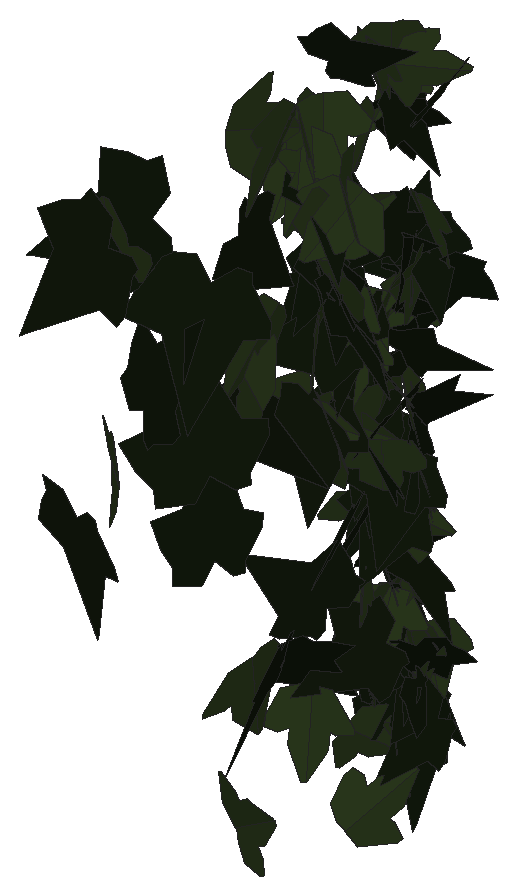
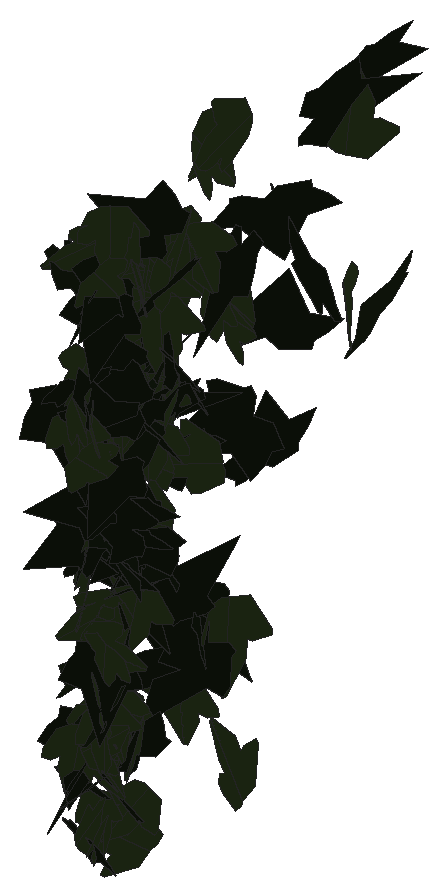
# SketchUp Ruby script. Lengths in inches.
U = 1.inch
M = Sketchup.active_model
def pt(a) = Geom::Point3d.new(a.map { |v| v * U })
def face(e, loops, mat)
  f = e.add_face(loops[0].map { |a| pt(a) })
  loops[1..].each { |l| e.add_face(l.map { |a| pt(a) }).erase! }
  f.material = f.back_material = mat if mat
  f
end
# faces: each face lists its corners as indices into pts; further lists are holes
def faces(e, pts, list, mat = nil) = list.each { |f| face(e, (f[0].is_a?(Array) ? f : [f]).map { |l| l.map { |i| pts[i] } }, mat) }
# xy, xz, yz: faces in a plane at the given z, y or x. An outline is a flat list of corners, or four numbers for a rectangle; further outlines are holes
def ring(l) = l.size == 4 ? [[l[0], l[1]], [l[2], l[1]], [l[2], l[3]], [l[0], l[3]]] : l.each_slice(2).to_a
def flat(e, list, mat, &to3) = list.each { |f| face(e, (f[0].is_a?(Array) ? f : [f]).map { |l| ring(l).map { |u, v| to3.(u, v) } }, mat) }
def xy(e, z, list, mat = nil) = flat(e, list, mat) { |x, y| [x, y, z] }
def xz(e, y, list, mat = nil) = flat(e, list, mat) { |x, z| [x, y, z] }
def yz(e, x, list, mat = nil) = flat(e, list, mat) { |y, z| [x, y, z] }
def lines(e, pts, list) = list.each { |a, b| e.add_line(pt(pts[a]), pt(pts[b])) }
# prism: a flat outline (further loops are holes) pulled along v
def prism(e, loops, v, mat = nil)
  f = face(e, loops, mat); d = Geom::Vector3d.new(v.map { |x| x * U })
  f.pushpull(f.normal.samedirection?(d) ? d.length : -d.length)
end
def box(e, o, s, mat = nil) = prism(e, [[o, [o[0] + s[0], o[1], o[2]], [o[0] + s[0], o[1] + s[1], o[2]], [o[0], o[1] + s[1], o[2]]]], [0, 0, s[2]], mat)
def at(x, y, z, deg = 0) = Geom::Transformation.translation(pt([x, y, z])) * Geom::Transformation.rotation(ORIGIN, Z_AXIS, deg.degrees)
def axes(o, x, y, z) = Geom::Transformation.new([*x, 0, *y, 0, *z, 0, *pt(o).to_a, 1])
def part(name) = M.definitions.add(name)
# library, detail: a bought-in or finely detailed component or shape, given as its bounding box
def library(name, o, s) = part(name).tap { |d| box(d.entities, o, s) }
def detail(e, o, s) = box(e.add_group.entities, o, s)
def put(e, d, t, mat = nil) = e.add_instance(d, t).tap { |i| i.material = mat if mat }
def group(e, t, mat = nil) = e.add_group.tap { |g| g.transformation = t; g.material = mat if mat }.entities
root = M.entities
M.materials.add("efeu1").color = [18, 25, 13]
M.materials.add("efeu2").color = [43, 57, 29]
c1 = part("ivyleaf_9")
p = [[1.54,2.16,1.25],[1.36,2.04,1.19],[-0.21,0.99,0.68],[-0.71,1.11,0.82],[-0.85,0.86,0.67],[-0.8,0.17,0.21],
  [-0.9,-0.01,0.1],[-0.67,-0.16,-0.02],[-0.08,-0.08,-0.05],[-0.03,-0.6,-0.4],[0.65,-0.88,-0.66],[0.83,-0.6,-0.49],
  [1.29,-0.42,-0.43],[1.8125,-0.07,-0.26],[1.21,0.44,0.15]]
faces(c1.entities,p,[[0,1,2,3,4,5,6,7,8,9,10,11,12,13,14]],"efeu1")
c2 = part("ivyleaf_10")
p = [[0,0.5,-0.03],[-0.0625,2.02,-0.43],[-0.19,2.01,-0.46],[-0.54,1.05,-0.29],[-0.52,0.625,-0.18],[-0.83,0.76,-0.28],
  [-1.16,0.64,-0.33],[-1.15,0.33,-0.24],[-0.77,-0.39,0.02],[-0.3,-0.51,0.16],[0.04,-0.48,0.23],[-0.02,2.01,-0.4375],
  [-0.06,2.01,-0.43],[0.04,-0.49,0.23],[0.67,-0.49,0.14],[1.38,0.36,-0.2],[1.375,0.51,-0.24],[0.81,0.65,-0.19],
  [0.62,0.59,-0.15],[0.6,1.09,-0.28],[0.5,1.23,-0.31]]
faces(c2.entities,p,[[0,1,2,3,4,5,6,7,8,9,10],[11,12,0,13,14,15,16,17,18,19,20]],"efeu2")
put(root,c1,axes([600.29,122.28,205.0625],[-0.40214,-0.86547,0.79158],[-0.29941,-0.73333,-0.9539],[1.13401,-0.50053,0.02885]))
put(root,c1,axes([599.61,122.04,197.19],[0.37416,-1.0394,0.54489],[0.18019,-0.51425,-1.10469],[1.15965,0.41527,-0.00415]))
put(root,c2,axes([599.48,123.61,203.85],[-1.04539,-0.23981,-0.03283],[-0.02592,-0.03381,1.0722],[-0.24065,1.04536,0.02715]))
put(root,c1,axes([599.8,124.59,204.78],[-0.4061,-0.51323,1.09008],[-0.71546,-0.82283,-0.65395],[0.96943,-0.82227,-0.02599]))
put(root,c2,axes([599.92,123.1,198.16],[0.11898,-0.07677,-1.11055],[-0.50468,0.99178,-0.12263],[0.99222,0.51366,0.07079]))
put(root,c1,axes([599.42,125.05,199.12],[-0.38662,0.62953,0.98563],[0.52664,-0.83317,0.73873],[1.04423,0.65328,-0.00764]))
put(root,c1,axes([600.54,126.14,202.38],[-0.56082,-1.10055,-0.27464],[0.12948,0.24226,-1.23519],[1.12688,-0.57555,0.00524]))
put(root,c1,axes([600.91,125.61,197.57],[-1.08701,-0.50646,0.39007],[0.35078,0.17072,1.19918],[-0.53442,1.14219,-0.00628]))
put(root,c1,axes([600.0625,126.9375,194.27],[-0.55763,-0.72017,0.76162],[0.45928,0.6076,0.91079],[-0.94222,0.72239,-0.00679]))
put(root,c2,axes([600.47,128.45,200.39],[0.01538,-0.78988,0.75027],[0.16421,-0.74009,-0.78253],[1.07696,0.12412,0.1086]))
put(root,c2,axes([601.02,127.48,198.9],[0.41463,0.06343,1.02926],[-1.00362,0.27973,0.38706],[-0.23695,-1.0738,0.16163]))
put(root,c2,axes([600.41,129.18,205.64],[0.32115,-0.86475,0.72869],[0.27952,-0.6733,-0.9222],[1.09574,0.42521,0.02168]))
put(root,c2,axes([600.11,128.07,205.86],[-0.05062,0.34907,1.048],[-0.21433,1.02606,-0.35211],[-1.08361,-0.21925,0.02069]))
put(root,c1,axes([600.19,129.29,190.26],[-0.59416,0.49067,-0.79124],[0.60187,-0.51371,-0.77052],[-0.71033,-0.84569,0.00897]))
put(root,c2,axes([599.6875,128.875,189.97],[-0.18213,-1.09237,-0.28856],[0.06624,0.28145,-1.1073],[1.1279,-0.19292,0.01843]))
put(root,c2,axes([598.9,129.44,184.95],[-0.61979,0.09958,0.90641],[0.88887,-0.1786,0.62742],[0.20349,1.08343,0.02012]))
put(root,c1,axes([598.86,129.02,197.02],[0.01173,0.03628,-1.07188],[0.77163,0.7442,0.03363],[0.74487,-0.77151,-0.01796]))
put(root,c1,axes([599.46,128.74,202.27],[0.23467,-0.25278,-1.10903],[-0.75295,0.81426,-0.34492],[0.85259,0.78867,0.00065]))
put(root,c1,axes([600.34,130.91,191.14],[0.0883,0.12547,0.96249],[-0.86791,-0.42251,0.1347],[0.43458,-0.8693,0.07346]))
put(root,c2,axes([599.97,130.8,188.23],[0.93842,0.21066,0.08673],[0.08075,0.03621,-0.96161],[-0.21303,0.94172,0.01758]))
put(root,c1,axes([600.04,131.24,196.4375],[-0.26241,-0.95865,-0.10441],[0.0171,0.10356,-0.99385],[0.96416,-0.26275,-0.01079]))
put(root,c2,axes([599.83,131.42,198.6],[0.26887,-0.69444,-0.82511],[0.30965,-0.76485,0.74462],[-1.03304,-0.41,0.00844]))
put(root,c1,axes([599.58,130.23,189.68],[0.73691,0.68881,0.20241],[0.14714,0.139,-1.0087],[-0.70269,0.75145,0.00104]))
put(root,c2,axes([599.34,131.21,203.8],[0.85784,0.50845,-0.2865],[-0.25947,-0.12396,-0.9969],[-0.52276,0.89588,0.02466]))
put(root,c2,axes([599.02,130.84,196.27],[0.12564,0.11221,0.99196],[0.79248,0.59677,-0.16788],[-0.60707,0.80226,-0.01386]))
put(root,c2,axes([599.53,131.9375,203.08],[-0.19042,-0.68735,0.71283],[0.16668,-0.73778,-0.66688],[0.97611,-0.0081,0.25294]))
put(root,c1,axes([600.85,130.53,192.89],[0.02867,0.57602,0.83709],[-0.03466,0.83749,-0.57511],[-1.01553,-0.01232,0.04325]))
put(root,c2,axes([600.72,131.51,202.49],[0.83957,0.22222,-0.52805],[-0.52716,-0.06716,-0.86642],[-0.22432,0.98955,0.05978]))
put(root,c2,axes([600.84,130.91,195.56],[-0.20643,0.28788,-0.9157],[-0.60349,0.68944,0.3528],[0.74645,0.63702,0.03199]))
put(root,c1,axes([600.05,132.0625,198.14],[-0.55826,-0.20289,0.73166],[-0.575,-0.4801,-0.57186],[0.49585,-0.78516,0.16061]))
put(root,c2,axes([600.5,131.43,200.29],[-0.65167,0.00787,0.7069],[-0.70586,0.04597,-0.65122],[-0.03913,-0.96035,-0.02538]))
put(root,c1,axes([600.28,131.71,199.7],[0.61641,-0.76466,-0.13822],[-0.09561,0.10045,-0.98211],[0.77115,0.62368,-0.01128]))
put(root,c2,axes([600.81,131.29,203.0625],[-0.52648,0.64251,0.59147],[-0.4426,0.39906,-0.82746],[-0.75284,-0.68393,0.07284]))
put(root,c2,axes([600.01,131.3,201.55],[-0.22951,-0.39398,0.86214],[0.37413,0.77738,0.45484],[-0.87094,0.43776,-0.0318]))
put(root,c1,axes([599.58,132.09,200.17],[-0.84931,0.02372,-0.32348],[0.32168,-0.05452,-0.84858],[-0.04154,-0.90719,0.04254]))
put(root,c2,axes([599.19,131.6875,204.37],[-0.4125,0.83818,0.00581],[-0.00664,0.00321,-0.93417],[-0.83817,-0.41253,0.00454]))
put(root,c1,axes([599.38,132.27,202.59],[0.16473,-0.99684,0.05025],[0.00925,-0.04941,-1.01036],[0.99807,0.16498,0.00107]))
put(root,c1,axes([599.55,132.24,199.41],[0.02687,-0.00182,0.92759],[0.45453,-0.80891,-0.01476],[0.8086,0.45477,-0.02253]))
put(root,c2,axes([599.57,131.91,204.47],[0.40389,0.90655,-0.10831],[-0.01535,-0.11168,-0.99196],[-0.91287,0.40297,-0.03125]))
put(root,c1,axes([599.64,132.52,199.79],[0.03911,-0.90435,0.36839],[0.10492,-0.36266,-0.90142],[0.97085,0.07562,0.08257]))
put(root,c2,axes([599.22,132.24,199.34],[-0.41496,0.4921,-0.58637],[0.39965,-0.4296,-0.64335],[-0.65289,-0.57573,-0.02113]))
put(root,c2,axes([599.85,132.05,201.4375],[-0.84036,-0.47868,0.15039],[-0.1313,-0.07334,-0.96713],[0.48426,-0.85056,-0.00124]))
put(root,c1,axes([600.7,132.8,189.36],[-0.5334,-0.52045,0.56705],[-0.41321,-0.38843,-0.74519],[0.64937,-0.67468,-0.0084]))
put(root,c2,axes([599.85,132.28,199.2],[0.90625,0.11586,-0.09509],[-0.09566,-0.00159,-0.91356],[-0.1154,0.91122,0.0105]))
put(root,c1,axes([599.58,132.36,199.77],[0.59913,-0.673,0.08127],[0.05691,-0.05814,-0.90104],[0.6755,0.60181,0.00383]))
put(root,c1,axes([599.81,132.17,199.77],[0.73858,-0.38363,-0.39965],[-0.36134,0.17126,-0.83217],[0.41992,0.82213,-0.01314]))
put(root,c2,axes([600.07,132.96,191.26],[-0.16152,0.36295,-0.78469],[0.27515,-0.73518,-0.39669],[-0.81961,-0.31833,0.02147]))
put(root,c1,axes([599.12,132.67,199.02],[0.05441,-0.92264,-0.35375],[-0.03847,0.35204,-0.9241],[0.98738,0.06456,-0.01652]))
put(root,c2,axes([599.71,132.54,197.84],[0.93416,0.2815,0.13783],[0.12776,0.05369,-0.97554],[-0.28621,0.94274,0.01441]))
put(root,c1,axes([600.21,133.17,194.5],[0.19189,-0.53853,0.65934],[0.32679,-0.57751,-0.5668],[0.7861,0.37153,0.07467]))
put(root,c1,axes([599.65,133.14,198.43],[-0.64862,-0.3588,-0.63371],[0.69422,-0.04832,-0.6832],[0.21997,-0.90552,0.28756]))
put(root,c1,axes([599.59,132.67,198.18],[0.8984,-0.30679,-0.04604],[-0.04236,0.01842,-0.94933],[0.30732,0.89939,0.00374]))
put(root,c1,axes([600.1,132.97,192.8],[-0.48301,0.56114,-0.48838],[0.31628,-0.37215,-0.74039],[-0.67332,-0.57734,0.00257]))
put(root,c2,axes([600.58,133.01,194.71],[-0.73717,-0.56369,0.0175],[-0.01091,-0.01455,-0.92797],[0.56385,-0.73723,0.00493]))
put(root,c2,axes([599.96,133.1,203.78],[0.54369,-0.70143,-0.14586],[-0.09414,0.11158,-0.88745],[0.71023,0.55175,-0.00597]))
put(root,c2,axes([599.67,132.71,198.49],[0.35341,0.72649,0.45874],[0.22215,0.4019,-0.80762],[-0.82999,0.41691,-0.02083]))
put(root,c2,axes([599.08,132.92,195.09],[-0.00232,-0.11604,0.88659],[0.83251,0.32318,0.04447],[-0.32622,0.82559,0.1072]))
put(root,c1,axes([599.71,133.67,195.73],[-0.6971,-0.50232,-0.09959],[0.08375,0.05412,-0.85921],[0.5052,-0.70209,0.00502]))
put(root,c1,axes([600.28,134.02,192.59],[-0.42046,-0.76182,0.23058],[0.12105,-0.31894,-0.83304],[0.78669,-0.35809,0.25142]))
put(root,c1,axes([600.61,133.85,193.96],[-0.43627,-0.81677,-0.07874],[0.03248,0.07192,-0.92597],[0.81991,-0.43744,-0.00522]))
put(root,c1,axes([598.7,133.33,205.11],[0.25592,-0.16925,0.78761],[0.79166,-0.10019,-0.27877],[0.14917,0.82206,0.12818]))
put(root,c2,axes([599.99,133.65,195.81],[-0.03093,-0.93867,0.12798],[0.06415,-0.12983,-0.93673],[0.94518,-0.0219,0.06776]))
put(root,c2,axes([599.84,132.97,184.0625],[0.40359,0.32833,-0.75922],[0.55257,0.52161,0.51931],[0.61553,-0.68354,0.03161]))
put(root,c1,axes([600.19,133.875,193.77],[-0.8438,-0.27352,-0.27388],[0.28564,0.0033,-0.8833],[0.26122,-0.88713,0.08116]))
put(root,c1,axes([599.76,133.89,194.86],[-0.5729,-0.58997,-0.24336],[0.23416,0.1099,-0.81767],[0.59368,-0.61266,0.08767]))
put(root,c1,axes([599.21,133.35,194.99],[-0.15545,-0.29097,-0.85133],[0.38273,0.76049,-0.32981],[0.81422,-0.41302,-0.00751]))
put(root,c1,axes([600.24,134.29,200.78],[-0.03646,-0.17743,-0.81499],[0.31475,-0.75838,0.15102],[-0.77241,-0.30066,0.10001]))
put(root,c1,axes([599.67,134.12,190.8],[0.10877,-0.2713,0.72355],[0.23929,-0.68294,-0.29205],[0.73476,0.26257,-0.012]))
put(root,c2,axes([599.45,133.59,192.66],[-0.65667,-0.51773,-0.14253],[0.11472,0.0847,-0.83621],[0.5246,-0.6666,0.00445]))
put(root,c2,axes([599.5,133.51,188.375],[-0.63,0.48567,0.12202],[-0.09984,0.07034,-0.79546],[-0.49071,-0.63784,0.00519]))
put(root,c2,axes([599.48,133.46,188.51],[-0.04387,0.71046,0.37985],[-0.01729,0.37949,-0.7118],[-0.80545,-0.04684,-0.00541]))
put(root,c1,axes([600.32,133.67,195.38],[-0.38932,0.83839,-0.18068],[0.07813,-0.16292,-0.92437],[-0.85407,-0.39708,-0.0022]))
put(root,c1,axes([599.42,133.51,187.55],[-0.25987,-0.14346,0.74979],[0.67696,0.32277,0.29639],[-0.35283,0.72494,0.01642]))
put(root,c2,axes([600.06,134.08,198.74],[0.37075,-0.76465,0.08712],[0.03224,-0.08118,-0.84977],[0.76893,0.37209,-0.00637]))
put(root,c2,axes([599.32,133.55,186.08],[-0.30301,-0.41844,-0.62456],[0.35496,0.51396,-0.51655],[0.6627,-0.46662,-0.00889]))
put(root,c2,axes([600.39,134.67,199],[-0.06366,-0.21168,-0.86217],[0.03225,-0.86436,0.20984],[-0.88719,-0.01623,0.06949]))
put(root,c1,axes([600.27,134.42,198.97],[0.04073,0.36594,0.81738],[-0.11604,-0.80917,0.36805],[0.88801,-0.12252,0.0106]))
put(root,c2,axes([599.71,134.26,189.56],[0.74881,0.31888,-0.08648],[-0.08022,-0.03234,-0.81388],[-0.32051,0.75309,0.00167]))
put(root,c1,axes([601.05,134.48,186.59],[-0.85033,-0.00663,-0.06762],[0.06757,0.00571,-0.85034],[0.00706,-0.85299,-0.00517]))
put(root,c2,axes([599.32,134.1875,205.25],[-0.76261,0.3137,-0.01831],[0.01519,-0.01121,-0.8246],[-0.31387,-0.76275,0.00459]))
put(root,c1,axes([599.17,133.74,195.21],[0.07256,-0.04731,0.88135],[0.61773,0.63436,-0.0168],[-0.63042,0.61614,0.08498]))
put(root,c1,axes([598.98,134.23,199.69],[0.57802,0.2456,-0.55657],[0.46743,0.31206,0.62315],[0.38935,-0.73925,0.07815]))
put(root,c1,axes([599.66,134.08,193.57],[0.55372,-0.34271,-0.54],[-0.37232,0.40804,-0.64074],[0.52003,0.65705,0.11625]))
put(root,c1,axes([600.16,134.76,190.74],[0.32381,-0.80205,0.25688],[0.28037,-0.15685,-0.84316],[0.79414,0.38241,0.19293]))
put(root,c2,axes([599.51,134.6,189.66],[0.04383,-0.8983,0.03926],[0.00393,-0.03912,-0.89937],[0.89915,0.04396,0.00201]))
put(root,c2,axes([599.91,134.22,192.47],[-0.39795,-0.24697,-0.71748],[0.64815,0.31063,-0.46642],[0.39456,-0.75938,0.04255]))
put(root,c2,axes([599.67,134.52,205.6875],[-0.58566,-0.5761,-0.00496],[-0.00017,0.00724,-0.8215],[0.57612,-0.58563,-0.00528]))
put(root,c1,axes([599.79,134.15,186.33],[-0.7592,0.38194,-0.05315],[-0.05107,0.01674,0.84982],[0.38223,0.76087,0.00798]))
put(root,c1,axes([600.19,135.2,194.24],[-0.03026,-0.18239,0.77363],[0.02116,-0.7741,-0.18168],[0.79456,0.01366,0.0343]))
put(root,c2,axes([600.19,134.55,195.61],[-0.42249,0.7387,-0.06593],[0.0315,-0.05793,-0.85099],[-0.74097,-0.42366,0.00141]))
put(root,c2,axes([600.07,134.57,186.11],[-0.70454,0.05519,0.25441],[-0.25541,-0.00448,-0.70632],[-0.05038,-0.74905,0.02297]))
put(root,c2,axes([600.05,134.74,191.48],[0.18129,0.10389,-0.81011],[-0.81673,0.02684,-0.17933],[0.00372,0.82971,0.10723]))
put(root,c2,axes([600.58,134.44,193.66],[-0.63029,0.60536,0.23266],[-0.18011,0.14828,-0.87375],[-0.62302,-0.6553,0.01722]))
put(root,c1,axes([600.48,134.92,200.18],[-0.09764,-0.74613,-0.30074],[0.03717,0.29843,-0.75249],[0.8036,-0.10446,-0.00174]))
put(root,c2,axes([599.78,134.72,185.59],[-0.29934,0.72176,-0.12043],[0.04935,-0.1099,-0.78136],[-0.73007,-0.30336,-0.00344]))
put(root,c2,axes([600.22,134.67,188.9],[-0.80293,0.09467,0.08482],[-0.08454,0.00741,-0.80849],[-0.09493,-0.80737,0.00253]))
put(root,c1,axes([600.0625,135.41,186.79],[-0.27648,-0.6071,0.41467],[0.04866,-0.45716,-0.63686],[0.73359,-0.19848,0.19853]))
put(root,c2,axes([599.6875,135.26,199.11],[0.20336,-0.18768,0.75877],[0.59324,-0.47345,-0.2761],[0.50895,0.62685,0.01865]))
put(root,c1,axes([600.5,134.52,188.43],[0.54031,0.57065,-0.23637],[-0.17293,-0.16172,-0.78574],[-0.59296,0.56714,0.01377]))
put(root,c1,axes([600.05,135.21,185.25],[-0.46153,-0.26694,-0.56654],[0.60396,-0.0035,-0.49037],[0.16571,-0.73073,0.20931]))
put(root,c2,axes([599.87,135.36,185.51],[-0.12652,0.438,0.68865],[0.19838,-0.65947,0.45589],[0.79166,0.23526,-0.00418]))
put(root,c1,axes([599.67,134.79,203.7],[0.42774,-0.52925,-0.44356],[-0.27873,0.34504,-0.68049],[0.63179,0.51054,0.00008]))
put(root,c2,axes([599.98,135.01,188.05],[-0.51537,0.00072,0.61171],[-0.59465,-0.1882,-0.50077],[0.14348,-0.77741,0.12179]))
put(root,c1,axes([600.36,134.72,187.32],[0.4298,-0.39761,-0.54607],[-0.34158,0.43044,-0.58228],[0.58276,0.54556,0.06143]))
put(root,c2,axes([600.38,134.9375,200.78],[-0.67379,0.37104,-0.24239],[0.21859,-0.10549,-0.7691],[-0.38554,-0.70826,-0.01244]))
put(root,c1,axes([599.21,134.64,197.8],[0.5877,0.53097,-0.10963],[-0.08826,-0.06583,-0.79197],[-0.53494,0.5942,0.01022]))
put(root,c1,axes([599.8,134.83,199.05],[-0.61953,-0.11518,0.52343],[0.52436,0.03526,0.62838],[-0.11088,0.81028,0.04706]))
put(root,c1,axes([599.2,135.3,189.74],[0.4582,-0.59403,0.26107],[0.17657,-0.19339,-0.74993],[0.62438,0.49062,0.02049]))
put(root,c1,axes([600.9,135.03,204.3],[-0.47506,0.62159,-0.18102],[0.04525,-0.1921,-0.77838],[-0.64583,-0.47068,0.07862]))
put(root,c1,axes([600.8,134.93,199.34],[0.49093,0.60434,-0.63358],[-0.4006,-0.49086,-0.77861],[-0.77857,0.63363,0.00112]))
put(root,c2,axes([599.46,135.02,189.42],[0.60029,-0.55914,0.08912],[-0.04526,0.08209,0.81984],[-0.56438,-0.6013,0.02905]))
put(root,c2,axes([599.42,135.12,189.42],[-0.42402,-0.68987,-0.02072],[0.02148,0.01112,-0.80967],[0.68985,-0.42438,0.01248]))
put(root,c1,axes([599.62,134.74,191.09],[0.23574,0.80529,-0.13647],[-0.05112,-0.12721,-0.83898],[-0.81517,0.24086,0.01315]))
put(root,c2,axes([600.32,135.17,188.44],[-0.66419,-0.56052,-0.10699],[0.21119,-0.08893,-0.84514],[0.53012,-0.66685,0.20264]))
put(root,c2,axes([599.8,135.15,188.36],[-0.45581,0.0973,-0.58477],[-0.58172,0.06857,0.46485],[0.1141,0.73825,0.03389]))
put(root,c2,axes([599.33,135.42,204.33],[0.29057,0.57132,-0.45747],[-0.21686,-0.40289,-0.64091],[-0.69904,0.36247,0.00867]))
put(root,c2,axes([600.06,134.69,204.88],[-0.09699,-0.26119,-0.78817],[0.56866,0.55733,-0.25467],[0.60503,-0.56569,0.11301]))
put(root,c2,axes([599.79,135.46,198.02],[0.35588,0.38665,-0.56675],[-0.4688,-0.32911,-0.51891],[-0.50092,0.5827,0.08299]))
put(root,c2,axes([599.1,135.32,191.83],[0.72765,-0.10436,0.28946],[0.28954,-0.01936,-0.73481],[0.10416,0.78287,0.02042]))
put(root,c2,axes([600.1,135.45,199.66],[0.08697,-0.7589,0.20736],[0.0581,-0.20186,-0.76313],[0.78457,0.09908,0.03352]))
put(root,c1,axes([599.47,134.6,203.83],[0.22207,0.70084,0.35668],[0.1091,0.33959,-0.73519],[-0.77878,0.24742,-0.00129]))
put(root,c1,axes([599.67,134.91,196.46],[0.57204,0.07636,0.53214],[0.52767,0.06884,-0.57712],[-0.10281,0.77825,-0.00116]))
put(root,c1,axes([599.38,134.93,203.21],[0.51931,0.56766,-0.23417],[-0.14785,-0.18207,-0.76925],[-0.596,0.53978,-0.01321]))
put(root,c2,axes([600.36,135.3,198.96],[-0.72786,-0.25848,0.20137],[-0.18649,-0.07654,-0.77233],[0.26941,-0.75131,0.0094]))
put(root,c1,axes([600.35,134.65,195.0625],[0.39345,0.43574,0.57124],[0.34233,0.45891,-0.58584],[-0.63166,0.52012,0.03832]))
